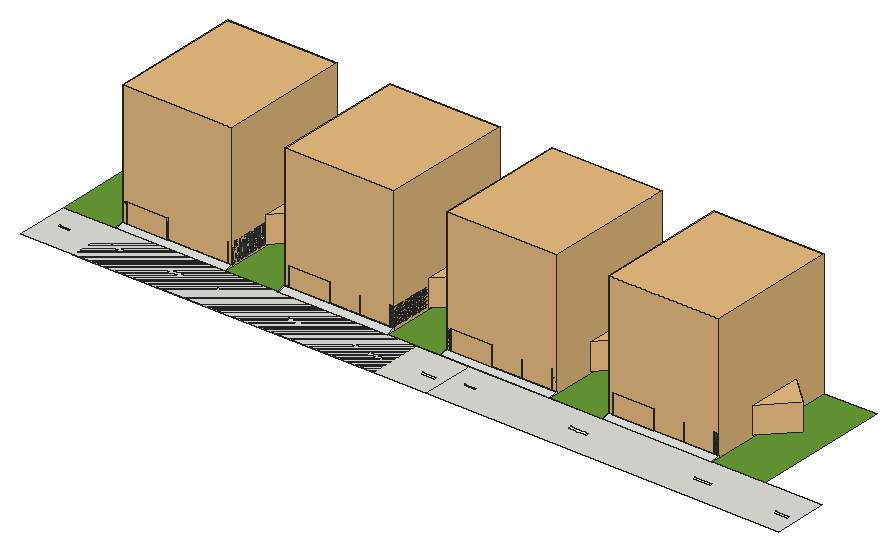
# SketchUp Ruby script. Lengths in inches.
U = 1.inch
M = Sketchup.active_model
def pt(a) = Geom::Point3d.new(a.map { |v| v * U })
def face(e, loops, mat)
  f = e.add_face(loops[0].map { |a| pt(a) })
  loops[1..].each { |l| e.add_face(l.map { |a| pt(a) }).erase! }
  f.material = f.back_material = mat if mat
  f
end
# faces: each face lists its corners as indices into pts; further lists are holes
def faces(e, pts, list, mat = nil) = list.each { |f| face(e, (f[0].is_a?(Array) ? f : [f]).map { |l| l.map { |i| pts[i] } }, mat) }
# xy, xz, yz: faces in a plane at the given z, y or x. An outline is a flat list of corners, or four numbers for a rectangle; further outlines are holes
def ring(l) = l.size == 4 ? [[l[0], l[1]], [l[2], l[1]], [l[2], l[3]], [l[0], l[3]]] : l.each_slice(2).to_a
def flat(e, list, mat, &to3) = list.each { |f| face(e, (f[0].is_a?(Array) ? f : [f]).map { |l| ring(l).map { |u, v| to3.(u, v) } }, mat) }
def xy(e, z, list, mat = nil) = flat(e, list, mat) { |x, y| [x, y, z] }
def xz(e, y, list, mat = nil) = flat(e, list, mat) { |x, z| [x, y, z] }
def yz(e, x, list, mat = nil) = flat(e, list, mat) { |y, z| [x, y, z] }
def lines(e, pts, list) = list.each { |a, b| e.add_line(pt(pts[a]), pt(pts[b])) }
# prism: a flat outline (further loops are holes) pulled along v
def prism(e, loops, v, mat = nil)
  f = face(e, loops, mat); d = Geom::Vector3d.new(v.map { |x| x * U })
  f.pushpull(f.normal.samedirection?(d) ? d.length : -d.length)
end
def box(e, o, s, mat = nil) = prism(e, [[o, [o[0] + s[0], o[1], o[2]], [o[0] + s[0], o[1] + s[1], o[2]], [o[0], o[1] + s[1], o[2]]]], [0, 0, s[2]], mat)
def at(x, y, z, deg = 0) = Geom::Transformation.translation(pt([x, y, z])) * Geom::Transformation.rotation(ORIGIN, Z_AXIS, deg.degrees)
def axes(o, x, y, z) = Geom::Transformation.new([*x, 0, *y, 0, *z, 0, *pt(o).to_a, 1])
def part(name) = M.definitions.add(name)
# library, detail: a bought-in or finely detailed component or shape, given as its bounding box
def library(name, o, s) = part(name).tap { |d| box(d.entities, o, s) }
def detail(e, o, s) = box(e.add_group.entities, o, s)
def put(e, d, t, mat = nil) = e.add_instance(d, t).tap { |i| i.material = mat if mat }
def group(e, t, mat = nil) = e.add_group.tap { |g| g.transformation = t; g.material = mat if mat }.entities
root = M.entities
M.materials.add("1480 AP K099 Starless Night-N").color = [54, 68, 77]
M.materials.add("BANANA_BIG_STVOL_1").color = [93, 83, 53]
M.materials.add("Color_000").color = [255, 255, 255]
M.materials.add("Material60").color = [234, 198, 157]
M.materials.add("POT_TEXTURE_1").color = [172, 172, 172]
M.materials.add("POT_TEXTURE_2").color = [160, 154, 144]
M.materials.add("[Color_009]").color = [33, 33, 33]
M.materials.add("[Color_A01]").color = [253, 112, 112]
M.materials.add("[Grass Dark Green]").color = [106, 157, 55]
M.materials.add("soil1").color = [68, 55, 47]
M.materials.add("white_concrete_pot1").color = [212, 211, 204]
M.materials.add("wood_1").color = [140, 119, 94]
c1 = part("Untitled")
xy(c1.entities,0,[[[158.81,26.5625,306.06,993.3125],[225.28,357.51,237.28,411.51],[239.71,931.55,251.46,972.3],[233.64,703.93,242.14,755.18],[222.04,66.5,231.29,100.5]]])
xy(c1.entities,0,[[222.04,66.5,231.29,100.5],[225.28,357.51,237.28,411.51],[233.64,703.93,242.14,755.18],[239.71,931.55,251.46,972.3]],"Color_000")
c2 = part("Group\#163")
xy(c2.entities,0,[[0,0,144,382]],"[Grass Dark Green]")
c3 = library("Modern Gate 1",[0,0,0],[118.11,1.97,78.74])
c4 = library("Window_Curtains2",[0,-81.89,0],[92,82.37,8.12])
c5 = part("Group\#33")
prism(c5.entities,[[[22.64,0,0],[0,0,0],[0,43.31,0],[22.64,43.31,0]],[[20.67,41.34,0],[1.97,41.34,0],[1.97,1.97,0],[20.67,1.97,0]]],[0,0,1.38])
c6 = part("Group\#34")
box(c6.entities,[0,0,0],[18.7,39.37,0.39])
c7 = part("2slidwin w fix bottom")
put(c7.entities,c5,axes([1.97,0,22.15],[1,0,0],[0,0,1.25],[0,-1,0]),"[Color_009]")
put(c7.entities,c6,axes([3.9375,-0.2,24.61],[1,0,0],[0,0,1.25],[0,-1,0]),"[Color_A01]")
g1 = group(c7.entities,at(0,-0.2,0),"[Color_009]")
prism(g1,[[[47.24,0,19.69],[0,0,19.69],[0,0,78.74],[47.24,0,78.74]],[[45.28,0,22.15],[45.28,0,76.28],[1.97,0,76.28],[1.97,0,22.15]]],[0,-3.15,0])
put(c7.entities,c5,axes([22.64,-1.38,22.15],[1,0,0],[0,0,1.25],[0,-1,0]),"[Color_009]")
put(c7.entities,c6,axes([24.61,-1.57,24.61],[1,0,0],[0,0,1.25],[0,-1,0]),"[Color_A01]")
c8 = library("Group\#12",[-312.76,2118.02,370.79],[80.37,61.43,57.53])
c9 = library("Group\#37",[-146.29,2044.53,349.125],[81,53.32,37.9])
c10 = library("Group\#85",[-236.03,2064.57,238.29],[378.97,266.89,1422.96])
c11 = library("Group\#21",[-392.38,2142.99,345.23],[79.77,60.6,39.05])
c12 = library("Group\#52",[-390.04,2074.71,363.78],[77.3,84.83,61.55])
c13 = library("Group\#25",[-389.63,2051.04,359.41],[56.81,81.38,37.86])
c14 = library("Group\#29",[-362.86,1963.26,351.01],[55.56,80.44,37.9])
c15 = library("Group\#36",[-200.52,1998.86,370.22],[77.15,68.38,35.39])
c16 = library("Group\#48",[-480.58,1843.32,11.96],[467.85,466.24,378.92])
c17 = library("Group\#22",[-433.57,2042.61,369.7],[71.79,72.8,37.85])
c18 = library("Group\#19",[-148.5,2084.1,354.63],[73.89,71.73,39.48])
c19 = library("Group\#63",[-372.4375,2154.5,374],[76.125,67.08,39.0625])
c20 = library("Group\#64",[-275.5,2156.34,352.11],[71.39,73.27,44.69])
c21 = library("Group\#42",[-143.56,2061.14,371.42],[79.79,63.19,51.3])
c22 = library("Group\#51",[-363.89,1895.22,354.63],[76.92,66.54,39.48])
c23 = library("Group\#44",[-145.08,2015.32,369.99],[82.29,54.05,37.9])
c24 = library("Group\#60",[-315.77,2202.04,371],[80.74,54.44,37.85])
c25 = library("Group\#53",[-419.21,1941.11,355.02],[73.1,71.21,39.06])
c26 = library("Group\#56",[-229.79,1894.04,351.01],[79.82,63.55,37.9])
c27 = library("Group\#70",[-234.26,2180.97,367.05],[50.63,74.65,43.95])
c28 = library("Group\#72",[-904.81,1865.01,156.3],[624.43,217.34,1227.7])
c29 = library("Group\#73",[-312.51,1611.52,263.78],[120.52,408.52,1275.1])
c30 = library("Group\#75",[-571.16,1736.08,232.33],[294.08,306.57,1438.75])
c31 = library("Group\#77",[-273.21,1593.22,47.51],[374.54,419.07,1416.6])
c32 = library("Group\#16",[-202.35,1900.5,372.29],[58.53,80.11,50.06])
c33 = library("Group\#24",[-432.01,1984.38,372.6875],[64.1,75.95,39.0625])
c34 = library("Group\#41",[-310.7,1952.62,354.63],[79.53,58.52,39.48])
c35 = library("Group\#23",[-374.28,1979.7,369.99],[51.81,82.66,37.9])
c36 = library("Group\#58",[-397.18,1916.74,372.44],[70.02,74.57,49.25])
c37 = library("Group\#66",[-236.3,2186.8,344.47],[79.26,62.91,39.06])
c38 = library("Group\#15",[-161.07,2117.49,373.61],[81.25,53.73,39.48])
c39 = library("Group\#71",[-431.9,1883.46,368.72],[373.65,376.39,18.61])
c40 = library("Group\#40",[-340.96,1970.4,361.28],[81.22,51.59,61.62])
c41 = library("Group\#46",[-272.7,1884.51,369.99],[80.39,55.87,37.9])
c42 = library("Group\#35",[-330.83,2117.69,370.2],[61.83,80.2,35.55])
c43 = library("Group\#69",[-366.3125,2177.8,359.41],[79.9,61.23,37.86])
c44 = library("Group\#28",[-435.875,2067.96,347.82],[58.32,80.53,38.29])
c45 = library("Group\#65",[-183.79,2161.45,371.25],[72.43,70.21,54.35])
c46 = library("Group\#76",[-208.23,2037.18,75.37],[621.09,225.61,1251.82])
c47 = library("Group\#79",[-675.58,1862.05,152.55],[378.81,196.01,1743.84])
c48 = library("Group\#80",[-257.06,2048.08,160.05],[394.6,177.93,1743.83])
c49 = library("Group\#82",[-344.84,1500.61,160.55],[176.35,551.19,1921.45])
c50 = library("Group\#83",[-231.77,1913.24,119.96],[448.93,143.84,1582.05])
c51 = library("Group\#84",[-616.67,2098.6,178.29],[331.19,111.16,1177.92])
c52 = library("Group\#78",[-527.15,2088.47,150.96],[267.01,328.12,1599.25])
c53 = library("Group\#87",[-792.12,2067.32,152.13],[549.56,259.52,1931.8])
c54 = library("Group\#88",[-281.17,2118.67,243.77],[133.23,408.71,1313.3])
c55 = part("Potted foliage plant")
g2 = group(c55.entities,at(904.81,-1500.61,-11.96),"white_concrete_pot1")
detail(g2,[-222.14,2117.95,372.07],[61.87,75.41,50.35])
put(c55.entities,c8,at(904.81,-1500.61,-11.96),"white_concrete_pot1")
g3 = group(c55.entities,at(904.81,-1500.61,-11.96),"white_concrete_pot1")
detail(g3,[-313.93,1881.02,351.21],[70.15,73.18,37.2])
g4 = group(c55.entities,at(904.81,-1500.61,-11.96),"white_concrete_pot1")
detail(g4,[-209.1,1970.26,378.89],[50.57,81.04,37.2])
put(c55.entities,c9,at(904.81,-1500.61,-11.96),"white_concrete_pot1")
put(c55.entities,c10,at(904.81,-1500.61,-11.96))
put(c55.entities,c11,at(904.81,-1500.61,-11.96),"white_concrete_pot1")
put(c55.entities,c12,at(904.81,-1500.61,-11.96),"white_concrete_pot1")
put(c55.entities,c13,at(904.81,-1500.61,-11.96),"white_concrete_pot1")
put(c55.entities,c14,at(904.81,-1500.61,-11.96),"white_concrete_pot1")
g5 = group(c55.entities,at(904.81,-1500.61,-11.96),"white_concrete_pot1")
detail(g5,[-129.49,1972.75,359.91],[55.59,80.76,37.2])
put(c55.entities,c15,at(904.81,-1500.61,-11.96),"white_concrete_pot1")
g6 = group(c55.entities,at(904.81,-1500.61,-11.96),"white_concrete_pot1")
detail(g6,[-333.13,1892.25,370.19],[61.39,79.4,37.2])
put(c55.entities,c16,at(904.81,-1500.61,-11.96),"POT_TEXTURE_1")
put(c55.entities,c17,at(904.81,-1500.61,-11.96),"white_concrete_pot1")
put(c55.entities,c18,at(904.81,-1500.61,-11.96),"white_concrete_pot1")
g7 = group(c55.entities,at(904.81,-1500.61,-11.96),"white_concrete_pot1")
detail(g7,[-270.91,2176.57,345.18],[52.11,82.01,38.29])
g8 = group(c55.entities,at(904.81,-1500.61,-11.96),"white_concrete_pot1")
detail(g8,[-195.71,2019.1875,371.11],[58.98,81.18,37.2])
g9 = group(c55.entities,at(904.81,-1500.61,-11.96),"white_concrete_pot1")
detail(g9,[-319.36,2078.81,339.18],[76.07,69.08,39.48])
put(c55.entities,c19,at(904.81,-1500.61,-11.96),"white_concrete_pot1")
put(c55.entities,c20,at(904.81,-1500.61,-11.96),"white_concrete_pot1")
g10 = group(c55.entities,at(904.81,-1500.61,-11.96),"white_concrete_pot1")
detail(g10,[-417.64,2112.53,369.82],[65.44,79.59,38.29])
put(c55.entities,c21,at(904.81,-1500.61,-11.96),"white_concrete_pot1")
put(c55.entities,c22,at(904.81,-1500.61,-11.96),"white_concrete_pot1")
put(c55.entities,c23,at(904.81,-1500.61,-11.96),"white_concrete_pot1")
g11 = group(c55.entities,at(904.81,-1500.61,-11.96),"white_concrete_pot1")
detail(g11,[-240.6,2054.85,378.89],[71.5,72.03,37.2])
put(c55.entities,c24,at(904.81,-1500.61,-11.96),"white_concrete_pot1")
put(c55.entities,c25,at(904.81,-1500.61,-11.96),"white_concrete_pot1")
put(c55.entities,c26,at(904.81,-1500.61,-11.96),"white_concrete_pot1")
g12 = group(c55.entities,at(904.81,-1500.61,-11.96),"white_concrete_pot1")
detail(g12,[-249.82,2117.53,359.91],[58.07,81.25,37.2])
put(c55.entities,c27,at(904.81,-1500.61,-11.96),"white_concrete_pot1")
put(c55.entities,c28,at(904.81,-1500.61,-11.96))
put(c55.entities,c29,at(904.81,-1500.61,-11.96))
put(c55.entities,c30,at(904.81,-1500.61,-11.96))
put(c55.entities,c31,at(904.81,-1500.61,-11.96))
g13 = group(c55.entities,at(904.81,-1500.61,-11.96),"white_concrete_pot1")
detail(g13,[-435.4375,2027.54,350.71],[78.74,62.6,37.86])
put(c55.entities,c32,at(904.81,-1500.61,-11.96),"white_concrete_pot1")
g14 = group(c55.entities,at(904.81,-1500.61,-11.96),"white_concrete_pot1")
detail(g14,[-173.8,2126.25,354.63],[80.17,60.53,39.48])
g15 = group(c55.entities,at(904.81,-1500.61,-11.96),"white_concrete_pot1")
detail(g15,[-222.96,2066.75,359.91],[63.77,78.21,37.2])
put(c55.entities,c33,at(904.81,-1500.61,-11.96),"white_concrete_pot1")
g16 = group(c55.entities,at(904.81,-1500.61,-11.96),"white_concrete_pot1")
detail(g16,[-183.125,1913.38,330.04],[66.78,77.69,39.48])
put(c55.entities,c34,at(904.81,-1500.61,-11.96),"white_concrete_pot1")
g17 = group(c55.entities,at(904.81,-1500.61,-11.96),"white_concrete_pot1")
detail(g17,[-152,1936.85,378.89],[64.46,79.76,37.2])
g18 = group(c55.entities,at(904.81,-1500.61,-11.96),"white_concrete_pot1")
detail(g18,[-284.65,1933.22,373.64],[80.83,55.23,37.2])
put(c55.entities,c35,at(904.81,-1500.61,-11.96),"white_concrete_pot1")
g19 = group(c55.entities,at(904.81,-1500.61,-11.96),"white_concrete_pot1")
detail(g19,[-263.49,1923.54,359.91],[75.98,66.75,37.2])
put(c55.entities,c36,at(904.81,-1500.61,-11.96),"white_concrete_pot1")
g20 = group(c55.entities,at(904.81,-1500.61,-11.96),"white_concrete_pot1")
detail(g20,[-167.97,1940.97,354.63],[66.78,77.7,39.48])
put(c55.entities,c37,at(904.81,-1500.61,-11.96),"white_concrete_pot1")
g21 = group(c55.entities,at(904.81,-1500.61,-11.96),"white_concrete_pot1")
detail(g21,[-214.75,1956.59,330.04],[66.78,77.69,39.48])
put(c55.entities,c38,at(904.81,-1500.61,-11.96),"white_concrete_pot1")
put(c55.entities,c39,at(904.81,-1500.61,-11.96),"white_concrete_pot1")
put(c55.entities,c40,at(904.81,-1500.61,-11.96),"white_concrete_pot1")
g22 = group(c55.entities,at(904.81,-1500.61,-11.96),"white_concrete_pot1")
detail(g22,[-282.5625,1934.21,389.56],[81.1,59.19,35.03])
put(c55.entities,c41,at(904.81,-1500.61,-11.96),"white_concrete_pot1")
g23 = group(c55.entities,at(904.81,-1500.61,-11.96),"white_concrete_pot1")
detail(g23,[-394.5,2036.48,359.91],[79.58,64.84,37.2])
put(c55.entities,c42,at(904.81,-1500.61,-11.96),"white_concrete_pot1")
put(c55.entities,c43,at(904.81,-1500.61,-11.96),"white_concrete_pot1")
put(c55.entities,c44,at(904.81,-1500.61,-11.96),"white_concrete_pot1")
put(c55.entities,c45,at(904.81,-1500.61,-11.96),"white_concrete_pot1")
put(c55.entities,c46,at(904.81,-1500.61,-11.96))
put(c55.entities,c47,at(904.81,-1500.61,-11.96))
put(c55.entities,c48,at(904.81,-1500.61,-11.96))
put(c55.entities,c49,at(904.81,-1500.61,-11.96))
put(c55.entities,c50,at(904.81,-1500.61,-11.96))
put(c55.entities,c51,at(904.81,-1500.61,-11.96))
put(c55.entities,c52,at(904.81,-1500.61,-11.96))
put(c55.entities,c53,at(904.81,-1500.61,-11.96))
put(c55.entities,c54,at(904.81,-1500.61,-11.96))
c56 = library("Group\#96",[-662.41,217.3,320.04],[397.32,658.3,1732.06])
c57 = library("Group\#98",[-299.2,181.55,262.58],[360.65,735.71,1258.34])
c58 = library("Group\#93",[-1038.76,656.55,345.34],[733.18,460.51,2065.7])
c59 = library("Group\#91",[-445.29,890.31,329.28],[284.3,304.08,2023.29])
c60 = library("Group\#94",[-733.48,439.625,202.64],[456.28,533.12,1536.78])
c61 = library("Group\#97",[-455.56,899.32,410.78],[341.21,610.33,1581.5])
c62 = library("Group\#90",[-516.34,626.77,-4.5625],[517.73,515.95,418.98])
c63 = library("Group\#95",[-249.24,914.85,310.18],[345.55,647.95,1307.93])
c64 = library("Group\#92",[-277.97,488.68,287.26],[362.84,405.94,1768.54])
c65 = library("Group\#89",[-468.76,669.89,380.1875],[424.36,427.47,41.99])
c66 = part("Potted broadleaf plant")
put(c66.entities,c56,at(1038.76,-181.55,4.5625))
put(c66.entities,c57,at(1038.76,-181.55,4.5625))
put(c66.entities,c58,at(1038.76,-181.55,4.5625))
put(c66.entities,c59,at(1038.76,-181.55,4.5625))
put(c66.entities,c60,at(1038.76,-181.55,4.5625))
put(c66.entities,c61,at(1038.76,-181.55,4.5625))
put(c66.entities,c62,at(1038.76,-181.55,4.5625),"POT_TEXTURE_1")
put(c66.entities,c63,at(1038.76,-181.55,4.5625))
put(c66.entities,c64,at(1038.76,-181.55,4.5625))
put(c66.entities,c65,at(1038.76,-181.55,4.5625),"soil1")
c67 = library("Group\#102",[-246.45,-349.05,558.47],[136.91,100.49,66.1])
c68 = library("Group\#105",[-264.68,-415.73,1484.11],[304.64,209.69,227.41])
c69 = library("Group\#112",[-357.04,-394.18,1447.05],[213.62,306.36,356.95])
c70 = library("Group\#100",[-447.02,-464.95,536.35],[343.73,346.24,39.39])
c71 = library("Group\#101",[-394.9,-448.99,911.74],[90.19,96.88,85.93])
c72 = library("Group\#111",[-424,-312.27,817.53],[158.81,108.06,136.45])
c73 = library("Group\#115",[-409.02,-515.05,915.53],[69.62,77.27,65.47])
c74 = library("Group\#119",[-548.25,-262.82,1459.54],[373.26,352.35,568])
c75 = library("Group\#129",[-492.14,-508.4,-4.15],[433.72,431.71,567.03])
c76 = library("Group\#122",[-293.78,-482.77,597.9],[158.75,112.78,159.87])
c77 = library("Group\#106",[-545.09,-386.51,922.3125],[300.25,219.65,227.33])
c78 = library("Group\#127",[-292.81,-667.38,1418.14],[215.17,356.07,188.87])
c79 = library("Group\#108",[-292.14,-288.9,1281.79],[169.55,204.34,203.36])
c80 = library("Group\#113",[-568.91,-444.37,1285.4],[307.6,179.39,277.93])
c81 = library("Group\#110",[-341.93,-403.49,744.8125],[64.83,96.32,132.15])
c82 = library("Group\#99",[-258.04,-282.68,604.05],[115.53,137.01,52.63])
c83 = library("Group\#107",[-304.79,-269.16,622.65],[82.06,111.89,102.57])
c84 = library("Group\#114",[-388.93,-514.39,838.93],[89.79,77.73,82.08])
c85 = library("Group\#116",[-295.03,-516.52,742.34],[68.71,141.75,78.67])
c86 = library("Group\#123",[-422.77,-235.4,843.61],[178.54,197.77,233.54])
c87 = library("Group\#117",[-498.98,-524.4,908.45],[120.83,107.95,112.98])
c88 = library("Group\#120",[-321.08,-139.66,1308.49],[285.55,393.29,221.53])
c89 = library("Group\#118",[-278.4,-571.99,1530.91],[311.57,345.77,423.62])
c90 = library("Group\#121",[-387.74,-136.11,1470.07],[230,321.58,230.27])
c91 = library("Group\#109",[-244.55,-305.59,1009.46],[103.13,76.81,77.34])
c92 = library("Group\#128",[-385.21,-446.52,494.02],[160.93,321.12,1142.36])
c93 = library("Group\#103",[-249.18,-250.59,980.93],[152.21,116.16,134.05])
c94 = library("Group\#104",[-438.92,-265.61,702.3],[171.52,146.16,133.5])
c95 = part("Potted broadleaf tree")
p = [[568.91,667.38,4.15],[569.91,667.38,4.15],[569.91,668.38,4.15]]
lines(c95.entities,p,[[0,1],[1,2],[2,0]])
put(c95.entities,c67,at(568.91,667.38,4.15))
put(c95.entities,c68,at(568.91,667.38,4.15))
put(c95.entities,c69,at(568.91,667.38,4.15))
put(c95.entities,c70,at(568.91,667.38,4.15),"soil1")
put(c95.entities,c71,at(568.91,667.38,4.15))
put(c95.entities,c72,at(568.91,667.38,4.15))
put(c95.entities,c73,at(568.91,667.38,4.15))
put(c95.entities,c74,at(568.91,667.38,4.15))
put(c95.entities,c75,at(568.91,667.38,4.15),"POT_TEXTURE_2")
put(c95.entities,c76,at(568.91,667.38,4.15))
put(c95.entities,c77,at(568.91,667.38,4.15))
put(c95.entities,c78,at(568.91,667.38,4.15))
put(c95.entities,c79,at(568.91,667.38,4.15))
put(c95.entities,c80,at(568.91,667.38,4.15))
put(c95.entities,c81,at(568.91,667.38,4.15))
put(c95.entities,c82,at(568.91,667.38,4.15))
put(c95.entities,c83,at(568.91,667.38,4.15))
put(c95.entities,c84,at(568.91,667.38,4.15))
put(c95.entities,c85,at(568.91,667.38,4.15))
put(c95.entities,c86,at(568.91,667.38,4.15))
put(c95.entities,c87,at(568.91,667.38,4.15))
put(c95.entities,c88,at(568.91,667.38,4.15))
put(c95.entities,c89,at(568.91,667.38,4.15))
put(c95.entities,c90,at(568.91,667.38,4.15))
put(c95.entities,c91,at(568.91,667.38,4.15))
put(c95.entities,c92,at(568.91,667.38,4.15),"wood_1")
put(c95.entities,c93,at(568.91,667.38,4.15))
put(c95.entities,c94,at(568.91,667.38,4.15))
c96 = library("Group\#137",[-640.625,-1318.37,287.11],[396.64,314.81,689.96])
c97 = library("Group\#132",[-513.94,-1201.2,195.17],[480.66,557.42,1160.08])
c98 = library("Group\#134",[-208.03,-1336.63,286.21],[381.72,484.79,1145.39])
c99 = library("Group\#140",[-619.83,-1636.3,288.9],[316.15,456.61,1171.28])
c100 = library("Group\#141",[-738.91,-1210.08,301],[426.4,388.88,1000.79])
c101 = library("Group\#143",[-208.33,-1511.76,297.04],[508.2,421.96,1258.76])
c102 = library("Group\#133",[-545.36,-1775.03,287.125],[412.21,432,920.68])
c103 = library("Group\#138",[-750.24,-1478.51,301.56],[423.84,451.05,998.69])
c104 = library("Group\#136",[-245.33,-1174.2,301.22],[356.02,306.31,608.34])
c105 = library("Group\#131",[-487.23,-1483.58,-4.71],[450.86,446.99,418.38])
c106 = library("Group\#145",[-445.7,-1606.55,154.18],[255.44,283.57,849.28])
c107 = library("Group\#146",[-390.1,-1177.12,195.59],[220.93,265.44,790.12])
c108 = library("Group\#148",[-480.32,-1333.42,295.8],[424.49,356.06,1482.77])
c109 = library("Group\#149",[-378.01,-1245.98,305.66],[422.15,474.55,1267.42])
c110 = library("Group\#135",[-163.65,-1622.09,292.29],[406.18,374.8,780.12])
c111 = library("Group\#144",[-384.8,-1640.99,300.61],[422.68,348.03,1297.96])
c112 = library("Group\#130",[-429.18,-1441.17,362.05],[345.84,348.28,45.35])
c113 = library("Group\#147",[-208.0625,-1498.77,286.27],[547.26,435.76,1075.6])
c114 = library("Group\#142",[-172.82,-1329.68,294.68],[502.85,397.72,955.79])
c115 = library("Group\#139",[-426.76,-1753.59,287.48],[479.67,412.35,1049.19])
c116 = part("Potted palm")
put(c116.entities,c96,at(750.24,1775.03,4.71))
put(c116.entities,c97,at(750.24,1775.03,4.71))
put(c116.entities,c98,at(750.24,1775.03,4.71))
put(c116.entities,c99,at(750.24,1775.03,4.71))
put(c116.entities,c100,at(750.24,1775.03,4.71))
put(c116.entities,c101,at(750.24,1775.03,4.71))
put(c116.entities,c102,at(750.24,1775.03,4.71))
put(c116.entities,c103,at(750.24,1775.03,4.71))
put(c116.entities,c104,at(750.24,1775.03,4.71))
put(c116.entities,c105,at(750.24,1775.03,4.71),"POT_TEXTURE_1")
put(c116.entities,c106,at(750.24,1775.03,4.71))
put(c116.entities,c107,at(750.24,1775.03,4.71))
put(c116.entities,c108,at(750.24,1775.03,4.71))
put(c116.entities,c109,at(750.24,1775.03,4.71))
put(c116.entities,c110,at(750.24,1775.03,4.71))
put(c116.entities,c111,at(750.24,1775.03,4.71))
put(c116.entities,c112,at(750.24,1775.03,4.71),"soil1")
put(c116.entities,c113,at(750.24,1775.03,4.71))
put(c116.entities,c114,at(750.24,1775.03,4.71))
put(c116.entities,c115,at(750.24,1775.03,4.71))
c117 = library("Group\#150",[-480.3,-2300.47,677.45],[398.14,398.43,28.25])
c118 = library("Group\#151",[-336.38,-2175.79,614.41],[133.99,147.1,560.64])
c119 = library("Group\#152",[-311.45,-2362.85,663.67],[597.01,322.07,1007.38])
c120 = library("Group\#153",[-330.26,-2159.14,612.04],[116.66,119.22,673.97])
c121 = library("Group\#154",[-667.53,-2111.4375,1071.74],[420.02,555.28,968.03])
c122 = library("Group\#155",[-328.97,-2115.58,1156.29],[117.86,119.42,695.38])
c123 = library("Group\#156",[-943.22,-2312.1875,967.59],[670.63,402.45,1245.73])
c124 = library("Group\#158",[-343.93,-2076.42,1024.91],[285.05,475.82,708.21])
c125 = library("Group\#157",[-568.09,-2386.9,-3.76],[573.62,569.18,700.28])
c126 = library("Group\#159",[-550.09,-2664.39,1031.96],[371.42,533.86,798])
c127 = library("Group\#160",[-308.37,-2556.11,869.35],[483.58,483.6,1385.8])
c128 = part("Potted broadleaf plant \#1")
put(c128.entities,c117,at(943.22,2664.39,3.76),"soil1")
put(c128.entities,c118,at(943.22,2664.39,3.76),"BANANA_BIG_STVOL_1")
put(c128.entities,c119,at(943.22,2664.39,3.76))
put(c128.entities,c120,at(943.22,2664.39,3.76),"BANANA_BIG_STVOL_1")
put(c128.entities,c121,at(943.22,2664.39,3.76))
put(c128.entities,c122,at(943.22,2664.39,3.76))
put(c128.entities,c123,at(943.22,2664.39,3.76))
put(c128.entities,c124,at(943.22,2664.39,3.76))
put(c128.entities,c125,at(943.22,2664.39,3.76),"POT_TEXTURE_2")
put(c128.entities,c126,at(943.22,2664.39,3.76))
put(c128.entities,c127,at(943.22,2664.39,3.76))
c129 = part("plants")
put(c129.entities,c55,at(-904.81,1500.61,11.96))
put(c129.entities,c66,at(-1038.76,181.55,-4.5625))
put(c129.entities,c95,at(-568.91,-667.38,-4.15))
put(c129.entities,c116,at(-750.24,-1775.03,-4.71))
put(c129.entities,c128,at(-943.22,-2664.39,-3.76))
put(c129.entities,c66,axes([-3769.8,7352.22,8291.06],[1,0,0],[0,1,0],[0,0,0.6]))
put(c129.entities,c66,axes([-4214.72,7065.25,4166.77],[1,0,0],[0,1,0],[0,0,0.726]))
c130 = library("Sliding windows",[337.77,-0.89,0.35],[154.53,8.85,122.84])
c131 = library("RANGE ROVER",[-63.71,-35.21,42.76],[182.88,182.88,64.08])
c132 = part("Bilal architect uae abu dhabi ")
put(c132.entities,c131,axes([104.22,-10.75,-48.75],[0.98727,0.57,0],[-0.57,0.98727,0],[0,0,1.14]),"Material60")
c133 = library("Group\#1",[0,0,0],[300,360,342])
c134 = part("Group\#161")
prism(c134.entities,[[[0,22,6],[0,22,0],[0,0,0]]],[300,0,0])
c135 = library("Group\#7",[0,-1,0],[111.5625,10,53])
c136 = part("Group")
box(c136.entities,[0,0,0],[12,55.4375,53])
c137 = part("Group\#6")
box(c137.entities,[0,0,0],[12,112.0625,53])
c138 = library("Group\#169",[0,0,0],[300,360,342])
c139 = library("Group\#173",[0,0,0],[300,360,342])
c140 = library("Group\#177",[0,0,0],[300,360,342])
put(root,c1,at(117.4375,306.06,0,-90))
put(root,c1,at(1084.1875,306.06,0,-90))
put(root,c1,at(-26.5625,306.06,0,-90))
put(root,c2,at(444,147.25,0))
put(root,c2,at(888,147.25,0))
put(root,c2,at(1332,147.25,0))
put(root,c2,at(1776,147.25,0))
put(root,c2,at(0,147.25,0))
g24 = group(root,at(144,147.25,0))
put(g24,c3,axes([123.5625,23.61,6],[0.69,0,0],[0,1,0],[0,0,0.62598]))
g25 = group(g24,at(0,0,0))
put(g25,c4,axes([27.28,108.99,125.3],[1.07666,0,0],[0,0,1.45695],[0,-1,0]))
put(g25,c4,axes([27.28,108.99,234.88],[1.07666,0,0],[0,0,1.25],[0,-1,0]))
put(g25,c7,axes([31,96.35,106.84],[1.86267,0,0],[0,1.5,0],[0,0,1.63366]))
put(g25,c7,axes([31,96.35,-34],[1.86267,0,0],[0,1.5,0],[0,0,2.032]))
g26 = group(g25,at(0,0,0))
put(g26,c4,axes([153.16,165.62,248.4],[1.43304,0,0],[0,0,1.25],[0,-1,0]))
put(g26,c129,axes([79.375,49.36,6.15],[0,-0.0242,0],[0.0242,0,0],[0,0,0.03194]))
put(g26,c130,axes([-107.47,156.95,138.69],[0.783,0,0],[0,0.74,0],[0,0,0.89551]))
put(g26,c132,axes([309.43,294.48,5.875],[-0.2287,-0.9735,0],[-0.9735,0.2287,0],[0,0,1]))
put(g26,c133,at(0,22,0))
put(g26,c134,at(0,0,0))
put(g24,c135,at(12,22,6))
put(g24,c136,at(0,22,6),"1480 AP K099 Starless Night-N")
put(g24,c137,at(288,22,6),"1480 AP K099 Starless Night-N")
g27 = group(root,at(588,147.25,0))
put(g27,c3,axes([123.5625,23.61,6],[0.69,0,0],[0,1,0],[0,0,0.62598]))
g28 = group(g27,at(0,0,0))
put(g28,c4,axes([27.28,108.99,125.3],[1.07666,0,0],[0,0,1.45695],[0,-1,0]))
put(g28,c4,axes([27.28,108.99,234.88],[1.07666,0,0],[0,0,1.25],[0,-1,0]))
put(g28,c7,axes([31,96.35,106.84],[1.86267,0,0],[0,1.5,0],[0,0,1.63366]))
put(g28,c7,axes([31,96.35,-34],[1.86267,0,0],[0,1.5,0],[0,0,2.032]))
g29 = group(g28,at(0,0,0))
put(g29,c4,axes([153.16,165.62,248.4],[1.43304,0,0],[0,0,1.25],[0,-1,0]))
put(g29,c129,axes([79.375,49.36,6.15],[0,-0.0242,0],[0.0242,0,0],[0,0,0.03194]))
put(g29,c130,axes([-107.47,156.95,138.69],[0.783,0,0],[0,0.74,0],[0,0,0.89551]))
put(g29,c132,axes([309.43,294.48,5.875],[-0.2287,-0.9735,0],[-0.9735,0.2287,0],[0,0,1]))
put(g29,c138,at(0,22,0))
put(g29,c134,at(0,0,0))
put(g27,c135,at(12,22,6))
put(g27,c136,at(0,22,6),"1480 AP K099 Starless Night-N")
put(g27,c137,at(288,22,6),"1480 AP K099 Starless Night-N")
g30 = group(root,at(1032,147.25,0))
put(g30,c3,axes([123.5625,23.61,6],[0.69,0,0],[0,1,0],[0,0,0.62598]))
g31 = group(g30,at(0,0,0))
put(g31,c4,axes([27.28,108.99,125.3],[1.07666,0,0],[0,0,1.45695],[0,-1,0]))
put(g31,c4,axes([27.28,108.99,234.88],[1.07666,0,0],[0,0,1.25],[0,-1,0]))
put(g31,c7,axes([31,96.35,106.84],[1.86267,0,0],[0,1.5,0],[0,0,1.63366]))
put(g31,c7,axes([31,96.35,-34],[1.86267,0,0],[0,1.5,0],[0,0,2.032]))
g32 = group(g31,at(0,0,0))
put(g32,c4,axes([153.16,165.62,248.4],[1.43304,0,0],[0,0,1.25],[0,-1,0]))
put(g32,c129,axes([79.375,49.36,6.15],[0,-0.0242,0],[0.0242,0,0],[0,0,0.03194]))
put(g32,c130,axes([-107.47,156.95,138.69],[0.783,0,0],[0,0.74,0],[0,0,0.89551]))
put(g32,c132,axes([309.43,294.48,5.875],[-0.2287,-0.9735,0],[-0.9735,0.2287,0],[0,0,1]))
put(g32,c139,at(0,22,0))
put(g32,c134,at(0,0,0))
put(g30,c135,at(12,22,6))
put(g30,c136,at(0,22,6),"1480 AP K099 Starless Night-N")
put(g30,c137,at(288,22,6),"1480 AP K099 Starless Night-N")
g33 = group(root,at(1476,147.25,0))
put(g33,c3,axes([123.5625,23.61,6],[0.69,0,0],[0,1,0],[0,0,0.62598]))
g34 = group(g33,at(0,0,0))
put(g34,c4,axes([27.28,108.99,125.3],[1.07666,0,0],[0,0,1.45695],[0,-1,0]))
put(g34,c4,axes([27.28,108.99,234.88],[1.07666,0,0],[0,0,1.25],[0,-1,0]))
put(g34,c7,axes([31,96.35,106.84],[1.86267,0,0],[0,1.5,0],[0,0,1.63366]))
put(g34,c7,axes([31,96.35,-34],[1.86267,0,0],[0,1.5,0],[0,0,2.032]))
g35 = group(g34,at(0,0,0))
put(g35,c4,axes([153.16,165.62,248.4],[1.43304,0,0],[0,0,1.25],[0,-1,0]))
put(g35,c129,axes([79.375,49.36,6.15],[0,-0.0242,0],[0.0242,0,0],[0,0,0.03194]))
put(g35,c130,axes([-107.47,156.95,138.69],[0.783,0,0],[0,0.74,0],[0,0,0.89551]))
put(g35,c132,axes([309.43,294.48,5.875],[-0.2287,-0.9735,0],[-0.9735,0.2287,0],[0,0,1]))
put(g35,c140,at(0,22,0))
put(g35,c134,at(0,0,0))
put(g33,c135,at(12,22,6))
put(g33,c136,at(0,22,6),"1480 AP K099 Starless Night-N")
put(g33,c137,at(288,22,6),"1480 AP K099 Starless Night-N")
